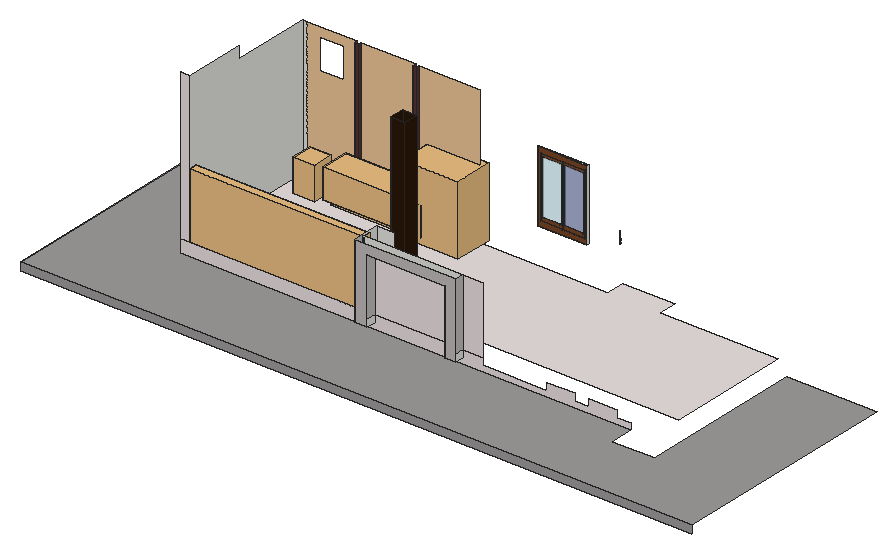
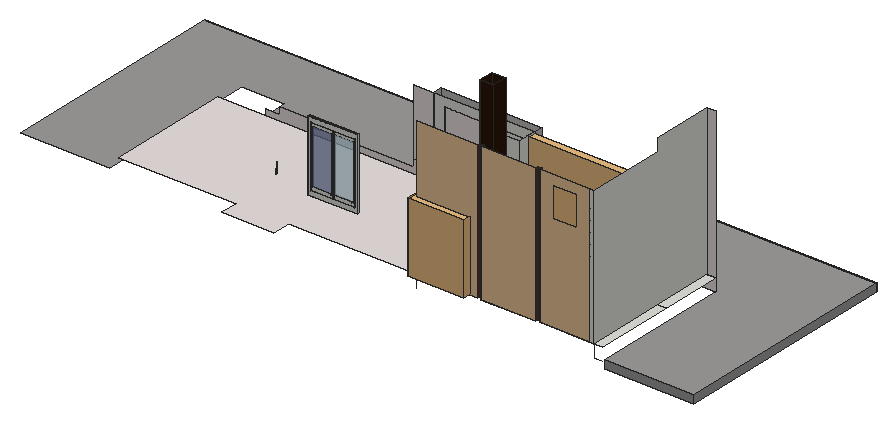
# SketchUp Ruby script. Lengths in inches.
U = 1.inch
M = Sketchup.active_model
def pt(a) = Geom::Point3d.new(a.map { |v| v * U })
def face(e, loops, mat)
  f = e.add_face(loops[0].map { |a| pt(a) })
  loops[1..].each { |l| e.add_face(l.map { |a| pt(a) }).erase! }
  f.material = f.back_material = mat if mat
  f
end
# faces: each face lists its corners as indices into pts; further lists are holes
def faces(e, pts, list, mat = nil) = list.each { |f| face(e, (f[0].is_a?(Array) ? f : [f]).map { |l| l.map { |i| pts[i] } }, mat) }
# xy, xz, yz: faces in a plane at the given z, y or x. An outline is a flat list of corners, or four numbers for a rectangle; further outlines are holes
def ring(l) = l.size == 4 ? [[l[0], l[1]], [l[2], l[1]], [l[2], l[3]], [l[0], l[3]]] : l.each_slice(2).to_a
def flat(e, list, mat, &to3) = list.each { |f| face(e, (f[0].is_a?(Array) ? f : [f]).map { |l| ring(l).map { |u, v| to3.(u, v) } }, mat) }
def xy(e, z, list, mat = nil) = flat(e, list, mat) { |x, y| [x, y, z] }
def xz(e, y, list, mat = nil) = flat(e, list, mat) { |x, z| [x, y, z] }
def yz(e, x, list, mat = nil) = flat(e, list, mat) { |y, z| [x, y, z] }
def lines(e, pts, list) = list.each { |a, b| e.add_line(pt(pts[a]), pt(pts[b])) }
# prism: a flat outline (further loops are holes) pulled along v
def prism(e, loops, v, mat = nil)
  f = face(e, loops, mat); d = Geom::Vector3d.new(v.map { |x| x * U })
  f.pushpull(f.normal.samedirection?(d) ? d.length : -d.length)
end
def box(e, o, s, mat = nil) = prism(e, [[o, [o[0] + s[0], o[1], o[2]], [o[0] + s[0], o[1] + s[1], o[2]], [o[0], o[1] + s[1], o[2]]]], [0, 0, s[2]], mat)
def at(x, y, z, deg = 0) = Geom::Transformation.translation(pt([x, y, z])) * Geom::Transformation.rotation(ORIGIN, Z_AXIS, deg.degrees)
def axes(o, x, y, z) = Geom::Transformation.new([*x, 0, *y, 0, *z, 0, *pt(o).to_a, 1])
def part(name) = M.definitions.add(name)
# library, detail: a bought-in or finely detailed component or shape, given as its bounding box
def library(name, o, s) = part(name).tap { |d| box(d.entities, o, s) }
def detail(e, o, s) = box(e.add_group.entities, o, s)
def put(e, d, t, mat = nil) = e.add_instance(d, t).tap { |i| i.material = mat if mat }
def group(e, t, mat = nil) = e.add_group.tap { |g| g.transformation = t; g.material = mat if mat }.entities
root = M.entities
M.materials.add("Generic").color = [243, 106, 23]
M.materials.add("Generic\#3").color = [43, 24, 10]
M.materials.add("Generic\#5").color = [191, 186, 186]
M.materials.add("Generic\#7").color = [87, 52, 52]
M.materials.add("Generic\#8").color = [235, 197, 151]
M.materials.add("Generic\#9").color = [233, 223, 223]
M.materials.add("Material \#1").color = [140, 140, 140]
M.materials.add("Wood Fine AI 03").color = [193, 179, 148]
M.materials.add("Wood Fine AI 03-CW").color = [193, 179, 148]
M.materials.add("[Granite Dark Gray]").color = [158, 155, 155]
M.materials.add("[Translucent_Glass_Safety]").color = [204, 235, 244]
M.materials["[Translucent_Glass_Safety]"].alpha = 0.5
M.materials.add("[Translucent_Glass_Sky_Reflection]").color = [125, 138, 183]
M.materials["[Translucent_Glass_Sky_Reflection]"].alpha = 0.52
M.materials.add("[Wood Veneer 01]").color = [120, 70, 37]
c1 = library("Raised potted plant",[1.65,0,0],[13.63,13.63,20.73])
c2 = library("Group\#3",[0,0,0],[146.75,6.73,55.76])
c3 = library("3dSolid\#17",[0,0,0],[103.74,27.56,5.91])
c4 = library("Group\#11",[0,0,0],[111.61,37.58,26.77])
c5 = part("Union")
xy(c5.entities,0,[[0,0,112.99,36.8125]],"Wood Fine AI 03-CW")
xy(c5.entities,1.38,[[1.38,0,111.61,35.43]],"Wood Fine AI 03-CW")
xy(c5.entities,25.59,[[0,0,1.38,0,1.38,35.43,0,36.8125],[111.61,0,112.99,0,112.99,36.8125,111.61,35.43]],"Wood Fine AI 03")
xy(c5.entities,25.59,[[1.38,35.43,111.61,35.43,112.99,36.8125,0,36.8125]],"Wood Fine AI 03-CW")
xz(c5.entities,0,[[0,0,1.38,1.38,1.38,25.59,0,25.59],[112.99,0,112.99,25.59,111.61,25.59,111.61,1.38]],"Wood Fine AI 03")
xz(c5.entities,0,[[0,0,112.99,0,111.61,1.38,1.38,1.38]],"Wood Fine AI 03-CW")
xz(c5.entities,35.43,[[1.38,1.38,111.61,25.59]],"Wood Fine AI 03")
xz(c5.entities,36.8125,[[0,0,112.99,25.59]],"Wood Fine AI 03")
yz(c5.entities,0,[[0,0,36.8125,25.59]],"Wood Fine AI 03")
yz(c5.entities,1.38,[[0,1.38,35.43,25.59]],"Wood Fine AI 03")
yz(c5.entities,111.61,[[0,1.38,35.43,25.59]],"Wood Fine AI 03")
yz(c5.entities,112.99,[[0,0,36.8125,25.59]],"Wood Fine AI 03")
c6 = library("Group3\#1",[-238.15,54.18,0],[46.4,43.96,56.68])
c7 = part("Sliding window")
xy(c7.entities,0,[[0,0,4.33,55.51]])
xy(c7.entities,2.76,[[0,2.76,2,27.76],[3.15,2.76,4.33,27.76],[0,27.76,0.82,52.76],[0.82,27.76,2.36,52.76],[2.36,27.76,4.33,52.76]])
xy(c7.entities,4.72,[[2,4.72,2.4,26.38],[2.76,4.72,3.15,26.38],[0.82,29.13,1.22,50.79],[1.97,29.13,2.36,50.79]])
xy(c7.entities,36.61,[[2,4.72,2.4,26.38],[2.76,4.72,3.15,26.38],[0.82,29.13,1.22,50.79],[1.97,29.13,2.36,50.79]])
xy(c7.entities,38.58,[[0,2.76,2,27.76],[3.15,2.76,4.33,27.76],[0,27.76,0.82,52.76],[0.82,27.76,2.36,52.76],[2.36,27.76,4.33,52.76]])
xy(c7.entities,41.34,[[0,0,4.33,55.51]])
xz(c7.entities,0,[[0,0,4.33,41.34]])
xz(c7.entities,2.76,[[0,2.76,2,38.58],[3.15,2.76,4.33,38.58]])
xz(c7.entities,4.72,[[2,4.72,2.4,36.61],[2.76,4.72,3.15,36.61]])
xz(c7.entities,26.38,[[2,4.72,2.4,36.61],[2.76,4.72,3.15,36.61]])
xz(c7.entities,27.76,[[0.82,2.76,2,38.58],[2,2.76,2.36,38.58],[2.36,2.76,3.15,38.58]])
xz(c7.entities,29.13,[[0.82,4.72,1.22,36.61],[1.97,4.72,2.36,36.61]])
xz(c7.entities,50.79,[[0.82,4.72,1.22,36.61],[1.97,4.72,2.36,36.61]])
xz(c7.entities,52.76,[[0,2.76,0.82,38.58],[0.82,2.76,2.36,38.58],[2.36,2.76,4.33,38.58]])
xz(c7.entities,55.51,[[0,0,4.33,41.34]])
yz(c7.entities,0,[[[0,0,55.51,41.34],[2.76,2.76,52.76,38.58]]])
yz(c7.entities,0.82,[[[27.76,2.76,52.76,38.58],[29.13,4.72,50.79,36.61]]])
yz(c7.entities,1.22,[[29.13,4.72,50.79,36.61]],"[Translucent_Glass_Sky_Reflection]")
yz(c7.entities,1.97,[[29.13,4.72,50.79,36.61]],"[Translucent_Glass_Sky_Reflection]")
yz(c7.entities,2,[[[2.76,2.76,27.76,38.58],[4.72,4.72,26.38,36.61]]])
yz(c7.entities,2.36,[[[27.76,2.76,52.76,38.58],[29.13,4.72,50.79,36.61]]],"[Wood Veneer 01]")
yz(c7.entities,2.4,[[4.72,4.72,26.38,36.61]],"[Translucent_Glass_Safety]")
yz(c7.entities,2.76,[[4.72,4.72,26.38,36.61]],"[Translucent_Glass_Safety]")
yz(c7.entities,3.15,[[[2.76,2.76,27.76,38.58],[4.72,4.72,26.38,36.61]]],"[Wood Veneer 01]")
yz(c7.entities,4.33,[[[0,0,55.51,41.34],[2.76,2.76,52.76,38.58]]],"[Wood Veneer 01]")
xy(root,-10.875,[[0,0,567.25,0,567.25,194.8125,491.875,194.8125,491.875,55,455.521,55,455.521,75.375,75.375,75.375,75.375,192.8125,0,192.8125]],"[Granite Dark Gray]")
xy(root,-6,[[228.293,67.75,238.793,75.375],[304.543,67.75,313.793,75.375]],"Generic\#5")
xy(root,0,[[75.375,75.375,82.8125,127.4375],[228.293,75.375,238.793,90.9375],[216.356,121.115,228.293,133.177],[75.375,127.4375,82.8125,194.8125]])
xy(root,0,[[[82.8125,75.375,228.293,75.375,228.293,90.9375,483.886,90.9375,483.886,194.8125,384.716,194.8125,384.716,210.0625,340.778,210.0625,340.778,194.8125,180.9375,194.8125,180.9375,192.5,177.9375,192.5,177.9375,194.8125,131.625,194.8125,131.625,192.5,128.625,192.5,128.625,194.8125,82.8125,194.8125],[216.356,121.115,228.293,133.177]]],"Generic\#9")
xy(root,40.624,[[347.812,199.268,347.812,199.557,347.848,199.557],[347.812,199.268,347.848,199.557,347.848,199.268]],"Material \#1")
xy(root,40.964,[[347.794,199.268,347.854,199.268,347.794,199.557],[347.854,199.268,347.854,199.557,347.794,199.557]],"Material \#1")
xz(root,0,[[0,-17.3125,567.25,-10.875]],"[Granite Dark Gray]")
xz(root,67.75,[[228.293,-6,238.793,-6,238.793,48.5625,304.543,48.5625,304.543,-6,313.793,-6,313.793,56.4375,228.293,56.4375]],"Generic\#5")
xz(root,75.375,[[228.293,-6,238.793,0],[304.543,-6,313.793,0],[228.293,0,228.293,56.4375,313.793,56.4375,313.793,0,304.543,0,304.543,48.5625,238.793,48.5625,238.793,0]])
xz(root,75.375,[[75.375,-10.875,455.521,-10.875,455.521,-6,443.584,-6,443.584,0,420.146,0,420.146,-6,408.209,-6,408.209,0,384.771,0,384.771,-6,330.78,-6,330.78,0,313.793,0,313.793,-6,304.543,-6,304.543,0,238.793,0,238.793,-6,228.293,-6,228.293,0,75.375,0],[75.375,0,82.8125,126],[238.793,0,304.543,48.5625],[313.793,0,330.78,56.4375]],"Generic\#9")
xz(root,90.9375,[[228.293,0,242.543,56.4375]])
xz(root,121.115,[[216.356,0,228.293,121.625]],"Generic\#3")
xz(root,133.177,[[216.356,0,228.293,121.625]],"Generic\#3")
xz(root,192.5,[[128.625,0,131.625,115.8125],[177.9375,0,180.9375,115.8125]],"Generic\#7")
xz(root,192.8125,[[0,-17.3125,75.375,-10.875]],"[Granite Dark Gray]")
xz(root,194.8125,[[82.8125,0,85.875,115.8125]])
xz(root,194.8125,[[[85.875,0,128.625,115.8125],[96.845,82.395,117.22,108.02]],[131.625,0,177.9375,115.8125],[180.9375,0,232.601,115.8125]],"Generic\#8")
xz(root,199.268,[[347.824,40.567,347.766,40.575,347.824,40.576],[347.824,40.567,347.824,40.576,347.879,40.583],[347.824,40.567,347.879,40.583,347.881,40.575],[347.766,40.575,347.713,40.598,347.768,40.583],[347.766,40.575,347.768,40.583,347.824,40.576],
  [347.881,40.575,347.879,40.583,347.93,40.605],[347.881,40.575,347.93,40.605,347.934,40.598],[347.768,40.583,347.713,40.598,347.717,40.605],[347.713,40.598,347.667,40.634,347.717,40.605],[347.934,40.598,347.93,40.605,347.974,40.64],
  [347.934,40.598,347.974,40.64,347.98,40.634],[347.717,40.605,347.667,40.634,347.673,40.64],[347.667,40.634,347.632,40.681,347.673,40.64],[347.98,40.634,347.974,40.64,348.008,40.685],[347.98,40.634,348.008,40.685,348.016,40.681],
  [347.673,40.64,347.632,40.681,347.639,40.685],[347.632,40.681,347.61,40.736,347.639,40.685],[348.016,40.681,348.008,40.685,348.03,40.738],[348.016,40.681,348.03,40.738,348.038,40.736],[347.639,40.685,347.61,40.736,347.618,40.738],
  [347.61,40.736,347.602,40.794,347.618,40.738],[348.038,40.736,348.03,40.738,348.037,40.794],[348.038,40.736,348.037,40.794,348.045,40.794],[347.618,40.738,347.602,40.794,347.61,40.794],[347.602,40.794,347.61,40.853,347.61,40.794],
  [347.61,40.794,347.61,40.853,347.618,40.851],[348.037,40.794,348.03,40.851,348.045,40.794],[348.045,40.794,348.03,40.851,348.038,40.853],[347.618,40.851,347.61,40.853,347.632,40.908],[347.618,40.851,347.632,40.908,347.639,40.904],
  [348.03,40.851,348.008,40.904,348.038,40.853],[348.038,40.853,348.008,40.904,348.016,40.908],[347.639,40.904,347.632,40.908,347.667,40.955],[347.639,40.904,347.667,40.955,347.673,40.949],[348.008,40.904,347.974,40.949,348.016,40.908],
  [348.016,40.908,347.974,40.949,347.98,40.955],[347.673,40.949,347.667,40.955,347.713,40.991],[347.673,40.949,347.713,40.991,347.717,40.984],[347.974,40.949,347.93,40.984,347.98,40.955],[347.98,40.955,347.93,40.984,347.934,40.991],
  [347.717,40.984,347.713,40.991,347.766,41.014],[347.717,40.984,347.766,41.014,347.768,41.006],[347.93,40.984,347.879,41.006,347.934,40.991],[347.934,40.991,347.879,41.006,347.881,41.014],[347.768,41.006,347.766,41.014,347.824,41.022],
  [347.768,41.006,347.824,41.022,347.824,41.013],[347.879,41.006,347.824,41.013,347.881,41.014],[347.824,41.013,347.824,41.022,347.881,41.014]],"Material \#1")
xz(root,199.277,[[347.824,40.059,347.701,40.12,347.947,40.12],[347.824,40.059,347.754,40.076,347.701,40.12],[347.824,40.059,347.788,40.064,347.754,40.076],[347.754,40.076,347.725,40.095,347.701,40.12],[347.947,40.12,347.544,40.756,347.63,40.635],
  [347.947,40.12,347.66,40.554,347.544,40.756],[347.701,40.12,347.666,40.53,347.666,40.536],[347.701,40.12,347.666,40.536,347.947,40.12],[347.701,40.12,347.67,40.184,347.666,40.53],[347.701,40.12,347.682,40.15,347.67,40.184],
  [347.947,40.12,347.714,40.565,347.767,40.546],[347.67,40.184,347.666,40.221,347.666,40.53],[347.66,40.554,347.657,40.56,347.544,40.756],[347.657,40.56,347.652,40.565,347.544,40.756],[347.652,40.565,347.598,40.622,347.544,40.756],
  [347.652,40.565,347.647,40.57,347.598,40.622],[347.647,40.57,347.621,40.594,347.598,40.622],[347.598,40.622,347.563,40.685,347.544,40.756],[347.598,40.622,347.579,40.652,347.563,40.685],[347.63,40.635,347.544,40.756,347.6,40.682],
  [347.6,40.682,347.544,40.756,347.582,40.736],[347.563,40.685,347.551,40.719,347.544,40.756],[347.582,40.736,347.544,40.756,347.575,40.794],[347.544,40.756,347.542,40.794,347.549,40.861],[347.544,40.756,347.549,40.861,347.604,40.975],
  [347.544,40.756,347.582,40.853,347.575,40.794],[347.544,40.756,347.604,40.975,347.582,40.853],[347.582,40.853,347.604,40.975,347.6,40.906],[347.549,40.861,347.571,40.921,347.604,40.975],[347.6,40.906,347.604,40.975,347.63,40.954],
  [347.63,40.954,347.604,40.975,347.668,40.993],[347.604,40.975,347.647,41.02,347.7,41.054],[347.604,40.975,347.7,41.054,347.824,41.083],[347.604,40.975,347.714,41.023,347.668,40.993],[347.604,40.975,347.824,41.083,347.714,41.023],
  [347.714,41.023,347.824,41.083,347.767,41.043],[347.767,41.043,347.824,41.083,347.824,41.049],[347.7,41.054,347.759,41.076,347.824,41.083]],"Material \#1")
xz(root,199.308,[[347.824,37.502,347.693,37.514,347.824,37.514],[347.693,37.514,347.571,37.548,347.696,37.526],[347.693,37.514,347.696,37.526,347.824,37.514],[347.696,37.526,347.571,37.548,347.575,37.56],[347.571,37.548,347.458,37.603,347.575,37.56],
  [347.575,37.56,347.458,37.603,347.464,37.614],[347.458,37.603,347.357,37.676,347.464,37.614],[347.464,37.614,347.357,37.676,347.365,37.686],[347.357,37.676,347.269,37.766,347.365,37.686],[347.365,37.686,347.269,37.766,347.279,37.774],
  [347.824,37.7,347.781,37.704,347.824,37.713],[347.781,37.704,347.74,37.716,347.783,37.717],[347.781,37.704,347.783,37.717,347.824,37.713],[347.74,37.716,347.702,37.734,347.744,37.728],[347.74,37.716,347.744,37.728,347.783,37.717],
  [347.744,37.728,347.702,37.734,347.708,37.745],[347.702,37.734,347.669,37.759,347.708,37.745],[347.708,37.745,347.669,37.759,347.677,37.768],[347.669,37.759,347.64,37.788,347.677,37.768],[347.269,37.766,347.201,37.863,347.279,37.774],
  [347.677,37.768,347.64,37.788,347.649,37.796],[347.279,37.774,347.201,37.863,347.212,37.87],[347.64,37.788,347.616,37.823,347.649,37.796],[347.649,37.796,347.616,37.823,347.627,37.829],[347.616,37.823,347.598,37.861,347.627,37.829],
  [347.627,37.829,347.598,37.861,347.61,37.866],[347.598,37.861,347.587,37.903,347.61,37.866],[347.201,37.863,347.144,37.986,347.212,37.87],[347.61,37.866,347.587,37.903,347.599,37.905],[347.212,37.87,347.144,37.986,347.156,37.99],
  [347.587,37.903,347.583,37.943,347.599,37.905],[347.599,37.905,347.583,37.943,347.595,37.943],[347.583,37.943,347.587,37.991,347.595,37.943],[347.595,37.943,347.587,37.991,347.599,37.989],[347.144,37.986,347.111,38.111,347.156,37.99],
  [347.599,37.989,347.587,37.991,347.598,38.033],[347.599,37.989,347.598,38.033,347.61,38.029],[347.156,37.99,347.111,38.111,347.123,38.113],[347.61,38.029,347.598,38.033,347.616,38.072],[347.61,38.029,347.616,38.072,347.627,38.065],
  [347.627,38.065,347.616,38.072,347.64,38.106],[347.627,38.065,347.64,38.106,347.649,38.098],[347.649,38.098,347.64,38.106,347.669,38.136],[347.649,38.098,347.669,38.136,347.677,38.126],[347.111,38.111,347.098,38.249,347.123,38.113],
  [347.123,38.113,347.098,38.249,347.111,38.25],[347.677,38.126,347.669,38.136,347.702,38.16],[347.677,38.126,347.702,38.16,347.708,38.149],[347.708,38.149,347.702,38.16,347.74,38.179],[347.708,38.149,347.74,38.179,347.744,38.167],
  [347.744,38.167,347.74,38.179,347.781,38.19],[347.744,38.167,347.781,38.19,347.783,38.178],[347.783,38.178,347.781,38.19,347.824,38.194],[347.783,38.178,347.824,38.194,347.824,38.181],[347.098,38.249,347.098,46.739,347.111,38.25],
  [347.111,38.25,347.098,46.739,347.111,46.738]],"Material \#1")
xz(root,199.339,[[347.824,40.539,347.759,40.548,347.824,40.548],[347.824,40.539,347.824,40.548,347.886,40.556],[347.824,40.539,347.886,40.556,347.888,40.548],[347.759,40.548,347.699,40.574,347.761,40.556],[347.759,40.548,347.761,40.556,347.824,40.548],
  [347.888,40.548,347.886,40.556,347.944,40.581],[347.888,40.548,347.944,40.581,347.948,40.574],[347.761,40.556,347.699,40.574,347.704,40.581],[347.699,40.574,347.648,40.614,347.704,40.581],[347.948,40.574,347.944,40.581,347.994,40.62],
  [347.948,40.574,347.994,40.62,348,40.614],[347.704,40.581,347.648,40.614,347.654,40.62],[347.648,40.614,347.608,40.667,347.654,40.62],[348,40.614,347.994,40.62,348.032,40.671],[348,40.614,348.032,40.671,348.039,40.667],
  [347.654,40.62,347.608,40.667,347.616,40.671],[347.608,40.667,347.583,40.728,347.616,40.671],[348.039,40.667,348.032,40.671,348.056,40.731],[348.039,40.667,348.056,40.731,348.064,40.728],[347.616,40.671,347.583,40.728,347.592,40.731],
  [347.583,40.728,347.575,40.794,347.592,40.731],[348.064,40.728,348.056,40.731,348.064,40.794],[348.064,40.728,348.064,40.794,348.072,40.794],[347.592,40.731,347.575,40.794,347.583,40.794],[347.575,40.794,347.583,40.86,347.583,40.794],
  [347.583,40.794,347.583,40.86,347.592,40.858],[348.064,40.794,348.056,40.858,348.072,40.794],[348.072,40.794,348.056,40.858,348.064,40.86],[347.592,40.858,347.583,40.86,347.608,40.922],[347.592,40.858,347.608,40.922,347.616,40.918],
  [348.056,40.858,348.032,40.918,348.064,40.86],[348.064,40.86,348.032,40.918,348.039,40.922],[347.616,40.918,347.608,40.922,347.648,40.975],[347.616,40.918,347.648,40.975,347.654,40.969],[348.032,40.918,347.994,40.969,348.039,40.922],
  [348.039,40.922,347.994,40.969,348,40.975],[347.654,40.969,347.648,40.975,347.699,41.015],[347.654,40.969,347.699,41.015,347.704,41.008],[347.994,40.969,347.944,41.008,348,40.975],[348,40.975,347.944,41.008,347.948,41.015],
  [347.704,41.008,347.699,41.015,347.759,41.041],[347.704,41.008,347.759,41.041,347.761,41.032],[347.944,41.008,347.886,41.032,347.948,41.015],[347.948,41.015,347.886,41.032,347.888,41.041],[347.761,41.032,347.759,41.041,347.824,41.049],
  [347.761,41.032,347.824,41.049,347.824,41.041],[347.886,41.032,347.824,41.041,347.888,41.041],[347.824,41.041,347.824,41.049,347.888,41.041]],"Material \#1")
xz(root,199.557,[[347.812,40.624,347.8,40.65,347.836,40.65],[347.812,40.624,347.836,40.65,347.848,40.624],[347.8,40.65,347.794,40.658,347.842,40.658],[347.8,40.65,347.842,40.658,347.836,40.65],[347.794,40.658,347.794,40.678,347.842,40.678],
  [347.794,40.658,347.842,40.678,347.842,40.658],[347.794,40.678,347.8,40.686,347.836,40.686],[347.794,40.678,347.836,40.686,347.842,40.678],[347.8,40.686,347.8,40.718,347.848,40.718],[347.8,40.686,347.848,40.718,347.836,40.686],
  [347.8,40.718,347.8,40.748,347.848,40.748],[347.8,40.718,347.848,40.748,347.848,40.718],[347.8,40.748,347.791,40.772,347.857,40.772],[347.8,40.748,347.857,40.772,347.848,40.748],[347.791,40.772,347.791,40.796,347.857,40.796],
  [347.791,40.772,347.857,40.796,347.857,40.772],[347.791,40.796,347.8,40.82,347.848,40.82],[347.791,40.796,347.848,40.82,347.857,40.796],[347.8,40.82,347.794,40.837,347.854,40.837],[347.8,40.82,347.854,40.837,347.848,40.82],
  [347.794,40.837,347.794,40.892,347.854,40.892],[347.794,40.837,347.854,40.892,347.854,40.837],[347.794,40.892,347.801,40.896,347.847,40.896],[347.794,40.892,347.847,40.896,347.854,40.892],[347.801,40.896,347.801,40.905,347.847,40.905],
  [347.801,40.896,347.847,40.905,347.847,40.896],[347.801,40.905,347.794,40.909,347.854,40.909],[347.801,40.905,347.854,40.909,347.847,40.905],[347.794,40.909,347.794,40.964,347.854,40.964],[347.794,40.909,347.854,40.964,347.854,40.909]],"Material \#1")
xz(root,199.588,[[347.824,40.059,347.754,40.076,347.788,40.064],[347.824,40.059,347.893,40.076,347.754,40.076],[347.754,40.076,347.666,40.53,347.67,40.184],[347.754,40.076,347.977,40.184,347.666,40.53],[347.754,40.076,347.67,40.184,347.701,40.12],
  [347.754,40.076,347.701,40.12,347.725,40.095],[347.701,40.12,347.67,40.184,347.682,40.15],[347.977,40.184,347.66,40.554,347.663,40.549],[347.977,40.184,347.663,40.549,347.665,40.543],[347.977,40.184,347.665,40.543,347.666,40.536],
  [347.67,40.184,347.666,40.53,347.666,40.221],[347.977,40.184,347.666,40.536,347.666,40.53],[347.981,40.221,347.63,40.635,347.66,40.554],[347.981,40.221,347.668,40.595,347.63,40.635],[347.981,40.221,347.714,40.565,347.668,40.595],
  [347.981,40.221,347.767,40.546,347.714,40.565],[347.66,40.554,347.544,40.756,347.657,40.56],[347.66,40.554,347.6,40.682,347.544,40.756],[347.66,40.554,347.63,40.635,347.6,40.682],[347.657,40.56,347.544,40.756,347.652,40.565],
  [347.652,40.565,347.544,40.756,347.598,40.622],[347.652,40.565,347.598,40.622,347.647,40.57],[347.647,40.57,347.598,40.622,347.621,40.594],[347.598,40.622,347.544,40.756,347.563,40.685],[347.598,40.622,347.563,40.685,347.579,40.652],
  [347.6,40.682,347.582,40.736,347.544,40.756],[347.563,40.685,347.544,40.756,347.551,40.719],[347.582,40.736,347.575,40.794,347.544,40.756],[347.544,40.756,347.549,40.861,347.542,40.794],[347.544,40.756,347.575,40.794,347.582,40.853],
  [347.544,40.756,347.582,40.853,347.6,40.906],[347.544,40.756,347.6,40.906,347.604,40.975],[347.544,40.756,347.604,40.975,347.549,40.861],[347.549,40.861,347.604,40.975,347.571,40.921],[347.6,40.906,347.63,40.954,347.604,40.975],
  [347.63,40.954,347.668,40.993,347.604,40.975],[347.604,40.975,347.668,40.993,347.714,41.023],[347.604,40.975,347.7,41.054,347.647,41.02],[347.604,40.975,347.714,41.023,347.824,41.083],[347.604,40.975,347.824,41.083,347.7,41.054],
  [347.714,41.023,347.767,41.043,347.824,41.083],[347.767,41.043,347.824,41.049,347.824,41.083],[347.7,41.054,347.824,41.083,347.759,41.076]],"Material \#1")
yz(root,0,[[0,-17.3125,192.8125,-10.875]],"[Granite Dark Gray]")
yz(root,82.8125,[[75.375,0,194.8125,0,194.8125,115.8125,127.4375,115.8125,127.4375,126,75.375,126]])
yz(root,128.625,[[192.5,0,194.8125,115.8125]],"Generic\#7")
yz(root,131.625,[[192.5,0,194.8125,115.8125]],"Generic\#7")
yz(root,177.9375,[[192.5,0,194.8125,115.8125]],"Generic\#7")
yz(root,180.9375,[[192.5,0,194.8125,115.8125]],"Generic\#7")
yz(root,216.356,[[121.115,0,133.177,121.625]],"Generic\#3")
yz(root,228.293,[[75.375,0,90.9375,56.4375]])
yz(root,228.293,[[121.115,0,133.177,121.625]],"Generic\#3")
yz(root,228.293,[[67.75,-6,75.375,56.4375]],"Generic\#5")
yz(root,238.793,[[67.75,-6,75.375,0]])
yz(root,238.793,[[67.75,0,75.375,48.5625]],"Generic\#5")
yz(root,304.543,[[67.75,-6,75.375,48.5625]],"Generic\#5")
yz(root,313.793,[[67.75,-6,75.375,0]])
yz(root,313.793,[[67.75,0,75.375,56.4375]],"Generic\#5")
yz(root,347.794,[[199.557,40.909,199.268,40.964,199.557,40.964]],"Material \#1")
yz(root,347.8,[[199.557,40.686,199.268,40.718,199.557,40.718]],"Material \#1")
p = [[347.741,199.308,37.876],[347.741,199.333,37.876],[347.722,199.34,37.849],[347.722,199.315,37.849],[347.743,199.34,37.83],[347.743,199.315,37.83],
  [347.769,199.34,37.816],[347.769,199.315,37.816],[347.787,199.333,37.843],[347.787,199.308,37.843],[347.803,199.33,37.867],[347.803,199.305,37.867],
  [347.757,199.305,37.899],[347.757,199.33,37.899],[347.845,199.305,38.028],[347.845,199.33,38.028],[347.891,199.33,37.995],[347.891,199.305,37.995],
  [347.861,199.308,38.052],[347.861,199.333,38.052],[347.907,199.333,38.019],[347.907,199.308,38.019],[347.925,199.34,38.045],[347.925,199.315,38.045],
  [347.904,199.34,38.065],[347.904,199.315,38.065],[347.879,199.34,38.078],[347.879,199.315,38.078],[347.797,199.268,40.654],[347.794,199.557,40.658],
  [347.8,199.557,40.65],[347.797,199.268,40.654],[347.8,199.557,40.65],[347.812,199.557,40.624],[347.812,199.268,40.624],[347.797,199.268,40.654],
  [347.791,199.268,40.784],[347.791,199.557,40.772],[347.8,199.557,40.748],[347.797,199.268,40.682],[347.794,199.557,40.678],[347.794,199.557,40.658],
  [347.797,199.268,40.654],[347.8,199.557,40.748],[347.795,199.268,40.76],[347.791,199.268,40.784],[347.797,199.268,40.682],[347.8,199.557,40.686],
  [347.794,199.557,40.678],[347.795,199.268,40.76],[347.8,199.557,40.748],[347.8,199.557,40.718],[347.8,199.557,40.718],[347.8,199.268,40.718],
  [347.795,199.268,40.76],[347.8,199.557,40.686],[347.797,199.268,40.682],[347.8,199.268,40.718],[347.795,199.268,40.808],[347.791,199.557,40.796],
  [347.791,199.557,40.772],[347.791,199.557,40.772],[347.791,199.268,40.784],[347.795,199.268,40.808],[347.791,199.557,40.796],[347.795,199.268,40.808],
  [347.797,199.268,40.828],[347.797,199.268,40.897],[347.794,199.557,40.892],[347.794,199.557,40.837],[347.794,199.557,40.837],[347.794,199.268,40.841],
  [347.797,199.268,40.897],[347.797,199.268,40.828],[347.8,199.557,40.82],[347.791,199.557,40.796],[347.794,199.268,40.841],[347.794,199.557,40.837],
  [347.8,199.557,40.82],[347.8,199.557,40.82],[347.797,199.268,40.828],[347.794,199.268,40.841],[347.794,199.557,40.909],[347.797,199.268,40.897],
  [347.794,199.268,40.964],[347.851,199.268,40.902],[347.854,199.557,40.892],[347.847,199.557,40.896],[347.797,199.268,40.897],[347.801,199.557,40.905],
  [347.801,199.557,40.896],[347.797,199.268,40.897],[347.794,199.557,40.909],[347.797,199.268,40.897],[347.794,199.557,40.892],[347.851,199.268,40.902],
  [347.847,199.557,40.905],[347.854,199.557,40.909],[347.851,199.268,40.902],[221.132,127.4375,115.8125],[221.132,127.4375,-3.9375],[75.375,194.8125,-10.875],
  [82.5,194.8125,-10.875],[232.601,194.8125,0],[232.601,194.8125,-10.875],[82.5,194.8125,0]]
faces(root,p,[[0,1,2],[2,3,0],[3,2,4],[4,5,3],[5,4,6],[6,7,5],[7,6,8],[8,9,7],
  [9,8,10],[10,11,9],[12,13,1],[1,0,12],[14,15,13],[13,12,14],[11,10,16],[16,17,11],
  [18,19,15],[15,14,18],[17,16,20],[20,21,17],[21,20,22],[22,23,21],[23,22,24],[24,25,23],
  [25,24,26],[26,27,25],[27,26,19],[19,18,27],[28,29,30],[31,32,33],[33,34,35],[36,37,38],
  [39,40,41],[41,42,39],[43,44,45],[46,47,48],[49,50,51],[52,53,54],[55,56,57],[58,59,60],
  [61,62,63],[64,65,66],[67,68,69],[70,71,72],[73,74,75],[76,77,78],[79,80,81],[82,83,84],
  [85,86,87],[88,89,90],[91,92,89],[93,90,94],[95,96,97],[98,87,96]],"Material \#1")
lines(root,p,[[99,100],[101,102],[103,104],[105,102]])
put(root,c1,axes([99.66,160.93,6.3125],[1.31013,0,0],[0,1.31013,0],[0,0,1.31013]),"Generic\#8")
put(root,c2,at(82.8125,75.375,0))
g1 = group(root,at(120.77,168,0))
put(g1,c3,axes([3.43,4.375,0],[0.74133,0,0],[0,0.61839,0],[0,0,0.86575]))
put(g1,c4,axes([0.51,0,5.32],[0.74133,0,0],[0,0.64313,0],[0,0,0.90783]),"Generic")
put(g1,c5,axes([0,1.51,5.11],[0.74133,0,0],[0,0.61839,0],[0,0,0.86575]))
put(root,c6,axes([430.55,128.05,0],[1.01951,0,0],[0,0.73674,0],[0,0,1.0388]))
put(root,c7,axes([280.76,197.03,29.46],[0,-0.28,0],[0.74759,0,0],[0,0,1.44992]))
